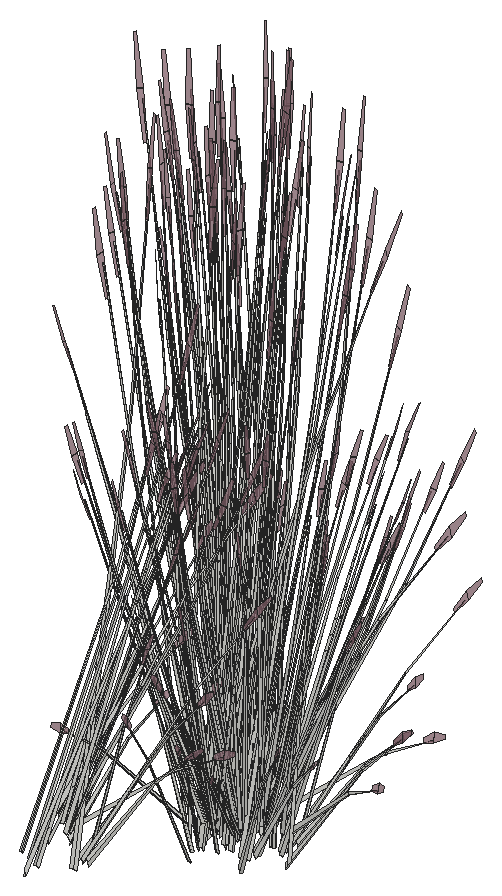
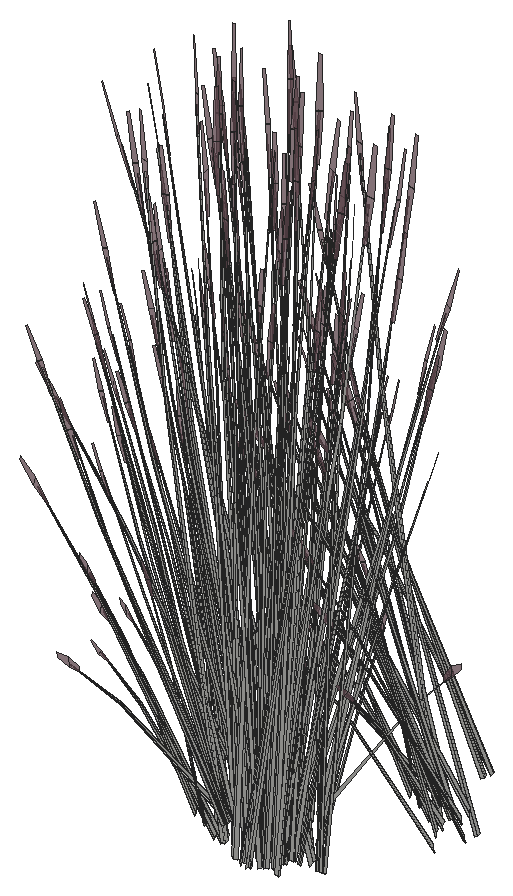
# SketchUp Ruby script. Lengths in inches.
U = 1.inch
M = Sketchup.active_model
def pt(a) = Geom::Point3d.new(a.map { |v| v * U })
def face(e, loops, mat)
  f = e.add_face(loops[0].map { |a| pt(a) })
  loops[1..].each { |l| e.add_face(l.map { |a| pt(a) }).erase! }
  f.material = f.back_material = mat if mat
  f
end
# faces: each face lists its corners as indices into pts; further lists are holes
def faces(e, pts, list, mat = nil) = list.each { |f| face(e, (f[0].is_a?(Array) ? f : [f]).map { |l| l.map { |i| pts[i] } }, mat) }
# xy, xz, yz: faces in a plane at the given z, y or x. An outline is a flat list of corners, or four numbers for a rectangle; further outlines are holes
def ring(l) = l.size == 4 ? [[l[0], l[1]], [l[2], l[1]], [l[2], l[3]], [l[0], l[3]]] : l.each_slice(2).to_a
def flat(e, list, mat, &to3) = list.each { |f| face(e, (f[0].is_a?(Array) ? f : [f]).map { |l| ring(l).map { |u, v| to3.(u, v) } }, mat) }
def xy(e, z, list, mat = nil) = flat(e, list, mat) { |x, y| [x, y, z] }
def xz(e, y, list, mat = nil) = flat(e, list, mat) { |x, z| [x, y, z] }
def yz(e, x, list, mat = nil) = flat(e, list, mat) { |y, z| [x, y, z] }
def lines(e, pts, list) = list.each { |a, b| e.add_line(pt(pts[a]), pt(pts[b])) }
# prism: a flat outline (further loops are holes) pulled along v
def prism(e, loops, v, mat = nil)
  f = face(e, loops, mat); d = Geom::Vector3d.new(v.map { |x| x * U })
  f.pushpull(f.normal.samedirection?(d) ? d.length : -d.length)
end
def box(e, o, s, mat = nil) = prism(e, [[o, [o[0] + s[0], o[1], o[2]], [o[0] + s[0], o[1] + s[1], o[2]], [o[0], o[1] + s[1], o[2]]]], [0, 0, s[2]], mat)
def at(x, y, z, deg = 0) = Geom::Transformation.translation(pt([x, y, z])) * Geom::Transformation.rotation(ORIGIN, Z_AXIS, deg.degrees)
def axes(o, x, y, z) = Geom::Transformation.new([*x, 0, *y, 0, *z, 0, *pt(o).to_a, 1])
def part(name) = M.definitions.add(name)
# library, detail: a bought-in or finely detailed component or shape, given as its bounding box
def library(name, o, s) = part(name).tap { |d| box(d.entities, o, s) }
def detail(e, o, s) = box(e.add_group.entities, o, s)
def put(e, d, t, mat = nil) = e.add_instance(d, t).tap { |i| i.material = mat if mat }
def group(e, t, mat = nil) = e.add_group.tap { |g| g.transformation = t; g.material = mat if mat }.entities
root = M.entities
M.materials.add("LightPink_Translucent").color = [144, 107, 117]
M.materials["LightPink_Translucent"].alpha = 0.75
c1 = part("blade")
p = [[2.15,0.21,22],[0,0.17,0],[0.09,0.45,0],[2.18,0.31,22],[2.29,0.31,22],[0.38,0.45,0],
  [2.48,0.24,33],[2.49,0.24,33],[2.48,0.22,33]]
faces(c1.entities,p,[[0,1,2,3],[4,5,2,3],[6,3,4,7],[8,0,3,6]])
c2 = part("seeds")
p = [[0.3,-0.1,1.38],[-0.01,-0.03,1.59],[-0.01,-0.03,0.03],[0.14,-0.07,-0.07],[0.29,-0.03,3],[0.15,0.01,3.11]]
faces(c2.entities,p,[[0,1,2,3],[1,0,4,5]],"LightPink_Translucent")
c3 = part("blade with seeds")
put(c3.entities,c1,at(0,0,0))
put(c3.entities,c2,axes([2.4,0.25,30.99],[1.5799,-0.05474,1.17369],[-0.12525,1.92788,0.29478],[-0.07173,-0.02425,1.56792]))
put(root,c3,axes([292.125,487.27,4.73],[0.32857,0.44488,0.0643],[-0.59916,0.21775,0.50621],[0.26412,-0.04296,0.77189]))
put(root,c3,axes([292.0625,487.11,4.73],[-0.25275,0.59491,0.48003],[-0.83094,-0.20343,0.3958],[0.32677,-0.03575,0.9933]))
put(root,c3,axes([291.625,482.97,4.68],[0.87941,0.16356,-0.51099],[-0.30143,0.56078,-0.3958],[0.08064,0.22578,0.97773]))
put(root,c3,axes([292.12,481.81,3.875],[-0.2045,-0.20949,1.71376],[0.94495,-0.17636,0.13857],[0.21357,0.32887,0.73262]))
put(root,c3,axes([289.7,486,2.06],[0.9306,0.10697,-0.62353],[-0.19638,0.65984,-0.16365],[0.27771,0.07995,1.37633]))
put(root,c3,axes([293.81,487.15,2.77],[-0.55274,0.10771,1.1486],[0.26018,-0.44517,0.84392],[0.29323,0.03046,0.25299]))
put(root,c3,axes([293.55,489.04,4.71],[-0.08089,-0.05712,1.77383],[0.17695,-0.61228,-0.16761],[0.31864,-0.03912,0.31391]))
put(root,c3,axes([291.3,482.86,4.98],[0.42698,0.53052,-0.71045],[-0.87893,0.29566,0.08574],[0.09984,0.25633,1.00501]))
put(root,c3,axes([292.85,488.53,3.93],[-0.17122,-0.54847,-0.03492],[0.80929,-0.12609,-0.15832],[0.169,0.03477,0.52218]))
put(root,c3,axes([290.75,488.51,5.03],[0.0479,-0.66354,-0.1216],[0.90696,0.01814,-0.67495],[0.3493,0.04609,1.02557]))
put(root,c3,axes([290.61,488.25,5.05],[-0.50902,-0.40851,0.35414],[0.58122,-0.38671,-0.4572],[0.29531,0.05884,0.87481]))
put(root,c3,axes([292.77,487.87,2.59],[-0.21545,-0.16047,1.43002],[0.28033,-0.53085,-0.30754],[0.43591,0.07191,0.61141]))
put(root,c3,axes([291.54,488.11,4.72],[0.19191,-0.01103,1.74944],[0.52639,-0.5069,-0.27667],[0.34136,0.06691,0.14031]))
put(root,c3,axes([290.8,488.19,4.98],[0.89428,0.01571,-0.71045],[-0.06006,0.66153,0.08574],[0.37886,0.06981,1.00501]))
put(root,c3,axes([297.4,493.71,4.72],[-0.13683,-0.09148,1.74944],[-0.91315,0.058,-0.27667],[-0.14574,-0.2188,0.14031]))
put(root,c3,axes([299.52,494.8,2.59],[-0.25429,0.13207,1.43002],[-0.76157,-0.23115,-0.30754],[0.14117,-0.28747,0.61141]))
put(root,c3,axes([298.36,495.26,4.98],[-0.42698,-0.53052,-0.71045],[0.87893,-0.29566,0.08574],[-0.09984,-0.25633,1.00501]))
put(root,c3,axes([292.26,486.85,2.375],[1.11865,0,0],[0,0.72922,-0.51607],[0,0.16609,1.63711]))
put(root,c3,axes([297.62,494.08,1.49],[-0.15005,0.02351,1.76342],[-0.82981,-0.26461,-0.26939],[0.01392,-0.22072,0.30037]))
put(root,c3,axes([291.33,488.46,4.53],[0.50902,0.40851,-0.35414],[-0.58122,0.38671,0.4572],[0.29531,0.05884,0.87481]))
put(root,c3,axes([291.07,488.62,4.73],[-0.04505,0.49615,0.0643],[-0.68022,-0.0136,0.50621],[0.26056,0.05192,0.77189]))
put(root,c3,axes([300.14,495.77,4.98],[0.02328,-0.60353,-0.71045],[0.98022,0.04053,0.08574],[0.10344,-0.25568,1.00501]))
put(root,c3,axes([291.14,488.46,4.73],[-0.65964,0.42992,0.48003],[-0.5689,-0.45657,0.3958],[0.30948,0.0793,0.9933]))
put(root,c3,axes([301.5,494.83,4.72],[-0.00864,-0.12985,1.74944],[-0.72937,-0.3753,-0.27667],[0.11277,-0.2275,0.14031]))
put(root,c3,axes([298.44,494.8,4.53],[0.2697,-0.50175,-0.35414],[0.78684,0.14635,0.4572],[-0.07215,-0.20201,0.87481]))
put(root,c3,axes([299.03,495.47,3.875],[-0.16657,0.22426,1.71376],[-0.69879,-0.4641,0.13857],[0.31524,-0.28926,0.73262]))
put(root,c3,axes([301.31,494.37,4.71],[-0.09085,0.04984,1.77383],[-0.89014,-0.16814,-0.16761],[-0.03222,-0.21748,0.31391]))
put(root,c3,axes([298.04,495.15,4.68],[-0.87941,-0.16356,-0.51099],[0.30143,-0.56078,-0.3958],[-0.08064,-0.22578,0.97773]))
put(root,c3,axes([298.58,493.74,2.77],[0.11476,0.38047,1.1486],[-0.63664,-0.21072,0.84392],[0.06851,-0.19481,0.25299]))
put(root,c3,axes([299.9375,495.57,4.68],[-0.64041,-0.4384,-0.51099],[0.67652,-0.38394,-0.3958],[0.09744,-0.22274,0.97773]))
put(root,c3,axes([289.51,487.42,3.875],[-0.3323,-0.11241,1.71376],[0.68769,-0.4716,0.13857],[0.42861,0.21275,0.73262]))
put(root,c3,axes([296.28,494.8,5.09],[0.99656,-0.1677,0.53763],[0.17295,0.65785,0.4433],[-0.23438,-0.19388,1.11249]))
put(root,c3,axes([298.54,494.92,4.73],[0.88151,0.17057,0.48003],[-0.30143,0.56078,0.3958],[-0.05297,-0.22053,0.9933]))
put(root,c3,axes([290.74,488.7,2.77],[-0.5037,-0.18761,1.1486],[0.6504,-0.19062,0.84392],[0.17543,0.16147,0.25299]))
put(root,c3,axes([298.79,495.12,5.03],[-0.87543,0.30377,-0.1216],[-0.4302,-0.53915,-0.67495],[-0.1155,-0.2272,1.02557]))
put(root,c3,axes([288.97,489.23,5.03],[0.53309,-0.55848,-0.1216],[0.77201,0.32175,-0.67495],[0.26836,0.15779,1.02557]))
put(root,c3,axes([300.61,495.8,5.03],[-0.98321,-0.03233,-0.1216],[0.02687,-0.61208,-0.67495],[0.0683,-0.23574,1.02557]))
put(root,c3,axes([300.54,495.41,4.53],[0.60531,-0.34352,-0.35414],[0.573,0.39225,0.4572],[0.08718,-0.19929,0.87481]))
put(root,c3,axes([298.77,494.88,4.73],[0.6592,-0.22175,0.0643],[0.32265,0.40436,0.50621],[-0.06366,-0.17825,0.77189]))
put(root,c3,axes([288.27,489.7,4.71],[0.00265,-0.07899,1.77383],[0.76665,-0.34851,-0.16761],[0.2663,0.12439,0.31391]))
put(root,c3,axes([290.88,489.39,1.49],[0.06518,-0.0942,1.76342],[0.82057,-0.27742,-0.26939],[0.24877,0.14358,0.30037]))
put(root,c3,axes([289.6,488.95,4.68],[0.88277,-0.1551,-0.51099],[0.15442,0.58737,-0.3958],[0.23711,0.16832,0.97773]))
put(root,c3,axes([296.51,494.94,4.73],[0.4066,-0.41448,0.0643],[0.57901,0.24131,0.50621],[-0.18719,-0.13288,0.77189]))
put(root,c3,axes([296.38,497.25,2.1],[-0.36739,-0.66907,-0.69835],[1.05831,-0.24096,-0.18329],[-0.04061,-0.22656,1.54149]))
put(root,c3,axes([301.3,495.2,1.49],[-0.1339,-0.0514,1.76342],[-0.34394,-0.57425,-0.26939],[0.23202,-0.15583,0.30037]))
put(root,c3,axes([290.82,489.55,2.67],[-0.57368,-0.02046,1.0506],[0.37886,-0.43461,0.58006],[0.22663,0.15441,0.8241]))
put(root,c3,axes([298.53,495.33,5.05],[-0.2697,0.50175,0.35414],[-0.78684,-0.14635,-0.4572],[-0.07215,-0.20201,0.87481]))
put(root,c3,axes([300.54,495.54,4.73],[0.63704,0.44518,0.48003],[-0.67652,0.38394,0.3958],[0.11751,-0.20886,0.9933]))
put(root,c3,axes([300.77,495.59,4.73],[0.73517,0.0304,0.0643],[-0.02016,0.45906,0.50621],[0.07693,-0.17585,0.77189]))
put(root,c3,axes([300.22,495.9,5.05],[-0.60531,0.34352,0.35414],[-0.573,-0.39225,-0.4572],[0.08718,-0.19929,0.87481]))
put(root,c3,axes([301.29,496.82,4.98],[0.4673,-0.51481,-0.71045],[0.81887,0.36587,0.08574],[0.27902,-0.18652,1.00501]))
put(root,c3,axes([296.24,495.32,2.375],[-0.55932,-0.6538,0],[0.93577,-0.36461,-0.51607],[0.21313,-0.08304,1.63711]))
put(root,c3,axes([301.27,496.58,4.68],[-0.22982,-0.59576,-0.51099],[0.87033,-0.10422,-0.3958],[0.24941,-0.16002,0.97773]))
put(root,c3,axes([288.94,488.5,2.59],[0.01579,-0.21629,1.43002],[0.75442,-0.24159,-0.30754],[0.23289,0.25887,0.61141]))
put(root,c3,axes([297.47,494.54,2.13],[-0.61821,0.37431,-0.03893],[-0.56645,-0.40995,-0.17649],[-0.03988,-0.11616,0.58215]))
put(root,c3,axes([301.68,497.01,5.03],[-0.82753,-0.35977,-0.1216],[0.47675,-0.52101,-0.67495],[0.2338,-0.18111,1.02557]))
put(root,c3,axes([294.22,497.15,2.02],[0,-0.65246,-0.49651],[1.00089,0,0],[0,-0.1486,1.57504]))
put(root,c3,axes([297,495.22,2.02],[0.83726,-0.32623,-0.49651],[0.50045,0.58498,0],[0.19069,-0.0743,1.57504]))
put(root,c3,axes([301.97,496.35,2.59],[-0.31959,-0.01933,1.43002],[-0.32741,-0.51843,-0.30754],[0.39262,-0.14666,0.61141]))
put(root,c3,axes([303.72,496.85,4.71],[-0.11685,-0.00496,1.77383],[-0.48522,-0.53096,-0.16761],[0.19486,-0.17458,0.31391]))
put(root,c3,axes([297.99,496.5625,2.06],[0.60257,-0.49041,-0.62353],[0.74854,0.44469,-0.16365],[0.24146,-0.12234,1.37633]))
put(root,c3,axes([302.34,495.4,2.77],[-0.29798,0.33213,1.1486],[-0.25612,-0.44624,0.84392],[0.24611,-0.11182,0.25299]))
put(root,c3,axes([301.91,496.65,4.53],[0.77872,-0.09325,-0.35414],[0.20563,0.53305,0.4572],[0.22316,-0.14318,0.87481]))
put(root,c3,axes([296.94,497.42,2.21],[0.43405,-0.58792,-0.44739],[0.90188,0.28295,0.21531],[0,-0.13553,1.43643]))
put(root,c3,axes([297.34,497.13,2.67],[-0.10425,-0.7445,-0.29095],[1.08575,-0.04502,-0.50002],[0.19119,-0.09917,1.59708]))
put(root,c3,axes([294.65,497.17,2.03],[0.62448,-0.40708,-0.30978],[0.62448,0.40708,0.30978],[0,-0.13112,1.38974]))
put(root,c3,axes([301.28,496.96,5.05],[-0.77872,0.09325,0.35414],[-0.20563,-0.53305,-0.4572],[0.22316,-0.14318,0.87481]))
put(root,c3,axes([296.83,497.91,2.67],[-1.00749,-0.31132,-0.29095],[0.48511,-0.65709,-0.50002],[-0.03166,-0.16133,1.59708]))
put(root,c3,axes([297.2,495.48,2.03],[0.83462,0.16144,-0.30978],[-0.21015,0.56852,0.30978],[0.16826,-0.06556,1.38974]))
put(root,c3,axes([301.98,496.875,4.73],[0.61415,0.2744,0.0643],[-0.35756,0.39076,0.50621],[0.1969,-0.12633,0.77189]))
put(root,c3,axes([301.81,496.76,4.73],[0.22187,0.60049,0.48003],[-0.87033,0.10422,0.3958],[0.25651,-0.14123,0.9933]))
put(root,c3,axes([304.16,497.49,4.72],[0.12414,-0.09938,1.74944],[-0.15889,-0.60963,-0.27667],[0.31148,-0.11559,0.14031]))
put(root,c3,axes([297.48,497.71,2.43],[1.00799,0.31623,0.24065],[-0.48511,0.65709,0.50002],[0,-0.15147,1.60543]))
put(root,c3,axes([297.09,498.6,2.4375],[0.23711,-0.77313,-0.23429],[1.12425,0.13477,0.51271],[-0.19645,-0.10677,1.5644]))
put(root,c3,axes([297.16,497.27,2.72],[-0.97146,0.04028,0.44739],[-0.08785,-0.66859,-0.21531],[0.17391,-0.06776,1.43643]))
put(root,c3,axes([294.65,497.76,2.48],[0,0.65246,0.49651],[-1.00089,0,0],[0,-0.1486,1.57504]))
put(root,c3,axes([301.71,498.41,5.03],[-0.45012,-0.59081,-0.1216],[0.79888,-0.29033,-0.67495],[0.33665,-0.07795,1.02557]))
put(root,c3,axes([301.67,497.91,4.68],[0.24236,-0.59349,-0.51099],[0.83094,0.20343,-0.3958],[0.33455,-0.05442,0.97773]))
put(root,c3,axes([300.36,495.49,2.375],[0.55932,-0.6538,0],[0.93577,0.36461,-0.51607],[0.21313,0.08304,1.63711]))
put(root,c3,axes([297.01,498.29,2.21],[-0.53742,-0.54764,-0.44739],[0.81403,-0.38564,0.21531],[-0.17391,-0.06776,1.43643]))
put(root,c3,axes([297.12,497.51,2.36],[0.38895,0.72959,0.45755],[-1.11135,0.2537,0.17955],[0.01358,-0.13406,1.58856]))
put(root,c3,axes([302.5625,498.07,1.98],[-0.57619,0.0783,1.41583],[-0.09171,-0.62326,0.08104],[0.40356,-0.09434,0.80566]))
put(root,c3,axes([303.61,497.52,2.26],[-0.55463,-0.41721,-0.06488],[0.60744,-0.38228,-0.29416],[0.17212,-0.02691,0.97024]))
put(root,c3,axes([296.93,498.09,2.72],[-0.43405,0.58792,0.44739],[-0.90188,-0.28295,-0.21531],[0,-0.13553,1.43643]))
put(root,c3,axes([298.52,497.58,2.21],[0,-0.75495,0],[1.11865,0,0],[0,0,1.79456]))
put(root,c3,axes([299.875,495.83,2.48],[-0.83726,-0.32623,0.49651],[0.50045,-0.58498,0],[0.19069,0.0743,1.57504]))
put(root,c3,axes([301.51,498.12,4.98],[0.78611,-0.28816,-0.71045],[0.4381,0.59317,0.08574],[0.37982,-0.06738,1.00501]))
put(root,c3,axes([297.99,497.1,2.36],[-0.74176,0.59212,0.45755],[-0.88124,-0.52269,0.17955],[0.17882,-0.05909,1.58856]))
put(root,c3,axes([298.8,498.16,2.3],[-0.83213,-0.56158,-0.06131],[0.83263,-0.56193,0],[-0.02906,-0.01961,1.75571]))
put(root,c3,axes([296.7,496.125,2.47],[-0.25843,0.64844,0.17642],[-0.9457,-0.1835,0.35086],[0.16336,-0.00316,1.60407]))
put(root,c3,axes([301.4,498.24,5.05],[-0.74348,-0.18202,0.35414],[0.21685,-0.53102,-0.4572],[0.29933,-0.04869,0.87481]))
put(root,c3,axes([296.3125,496.65,1.59],[-0.88056,0.26122,1.28929],[-0.28027,-0.74951,0.50096],[0.54072,0.01247,1.46642]))
put(root,c3,axes([298.68,496.85,2.62],[0.17258,-0.58229,0.1448],[0.84319,0.10108,-0.41347],[0.15345,0.05979,1.26744]))
put(root,c3,axes([297.22,498.23,2.36],[1.13071,0.13747,0.45755],[-0.23011,0.77639,0.17955],[-0.16524,-0.07497,1.58856]))
put(root,c3,axes([303.1875,497.67,1.49],[-0.04675,-0.09906,1.76342],[0.32428,-0.57943,-0.26939],[0.32711,-0.00833,0.30037]))
put(root,c3,axes([298.32,497,2.72],[-0.53742,-0.54764,0.44739],[0.81403,-0.38564,-0.21531],[0.17391,0.06776,1.43643]))
put(root,c3,axes([296.61,499.47,2.47],[0.96132,-0.17317,0.17642],[0.23737,0.64447,0.35086],[-0.08574,-0.0939,1.60407]))
put(root,c3,axes([298.59,497.03,2.67],[0.90324,-0.43318,-0.29095],[0.60064,0.61207,-0.50002],[0.22285,0.06216,1.59708]))
put(root,c3,axes([302.18,498.18,4.53],[0.74348,0.18202,-0.35414],[-0.21685,0.53102,0.4572],[0.29933,-0.04869,0.87481]))
put(root,c3,axes([300.87,495.88,2.02],[0.83726,0.32623,-0.49651],[-0.50045,0.58498,0],[0.19069,0.0743,1.57504]))
put(root,c3,axes([299.28,497.74,2.21],[1.00089,0,0],[0,0.67548,0],[0,0,1.78407]))
put(root,c3,axes([299.5625,496.16,2.47],[-0.96132,0.17317,0.17642],[-0.23737,-0.64447,0.35086],[0.08574,0.0939,1.60407]))
put(root,c3,axes([300.16,497.52,3.875],[-0.37107,0.01478,1.71376],[0.24616,-0.64047,0.13857],[0.5288,0.03961,0.73262]))
put(root,c3,axes([300.64,496.125,2.03],[0.21015,0.56852,-0.30978],[-0.83462,0.16144,0.30978],[0.16826,0.06556,1.38974]))
put(root,c3,axes([302.07,498.4,4.73],[0.32857,0.44488,0.0643],[-0.59916,0.21775,0.50621],[0.26412,-0.04296,0.77189]))
put(root,c3,axes([298.96,497.4,2.38],[-1.13071,-0.13747,0.49198],[0.23011,-0.77639,0.19306],[0.16524,0.07497,1.70813]))
put(root,c3,axes([302.01,498.24,4.73],[-0.25275,0.59491,0.48003],[-0.83094,-0.20343,0.3958],[0.32677,-0.03575,0.9933]))
put(root,c3,axes([298.05,499.32,2.2],[-0.29189,-0.56252,0],[0.83351,-0.19699,0],[0,0,1.54371]))
put(root,c3,axes([297.5,498.78,2.62],[-0.17258,0.58229,0.1448],[-0.84319,-0.10108,-0.41347],[-0.15345,-0.05979,1.26744]))
put(root,c3,axes([299.15,499.24,2.18],[0.93921,-0.22138,-0.19198],[0.33003,0.6377,0.00008],[0.10367,-0.02447,1.73897]))
put(root,c3,axes([299.47,499.5,2.47],[0.25843,-0.64844,0.17642],[0.9457,0.1835,0.35086],[-0.16336,0.00316,1.60407]))
put(root,c3,axes([299.26,498.03,2.21],[0.62448,0.42144,0],[-0.62448,0.42144,0],[0,0,1.69266]))
put(root,c3,axes([300.95,497.85,2.47],[-0.70288,-0.47526,0.17642],[0.70832,-0.46097,0.35086],[-0.07763,0.09706,1.60407]))
put(root,c3,axes([299.65,497.13,2.06],[0.9306,0.10697,-0.62353],[-0.19638,0.65984,-0.16365],[0.27771,0.07995,1.37633]))
put(root,c3,axes([303.76,498.28,2.77],[-0.55274,0.10771,1.1486],[0.26018,-0.44517,0.84392],[0.29323,0.03046,0.25299]))
put(root,c3,axes([297.85,499.57,2.2],[-0.90188,-0.29293,0],[0.43405,-0.60866,0],[0,0,1.62707]))
put(root,c3,axes([298.6,498.79,2.46],[-0.87356,-0.52515,-0.25192],[0.73507,-0.5897,0.5513],[-0.23523,0.06143,1.68216]))
put(root,c3,axes([296.3,499.8,2.48],[0.83726,0.32623,0.49651],[-0.50045,0.58498,0],[-0.19069,-0.0743,1.57504]))
put(root,c3,axes([299.25,497.54,2.72],[0.43405,-0.58792,0.44739],[0.90188,0.28295,-0.21531],[0,0.13553,1.43643]))
put(root,c3,axes([303.5,500.17,4.71],[-0.08089,-0.05712,1.77383],[0.17695,-0.61228,-0.16761],[0.31864,-0.03912,0.31391]))
put(root,c3,axes([299.08,497.875,2.29],[0,0.75458,-0.05637],[-1.11865,0,0],[0,0.02371,1.79368]))
put(root,c3,axes([299.16,497.34,2.21],[0.53742,0.54764,-0.44739],[-0.81403,0.38564,0.21531],[0.17391,0.06776,1.43643]))
put(root,c3,axes([302.8,499.66,3.93],[-0.17122,-0.54847,-0.03492],[0.80929,-0.12609,-0.15832],[0.169,0.03477,0.52218]))
put(root,c3,axes([300.7,499.64,5.03],[0.0479,-0.66354,-0.1216],[0.90696,0.01814,-0.67495],[0.3493,0.04609,1.02557]))
put(root,c3,axes([301.53,497.87,2.48],[0,-0.65246,0.49651],[1.00089,0,0],[0,0.1486,1.57504]))
put(root,c3,axes([299.02,498.36,2.72],[0.97146,-0.04028,0.44739],[0.08785,0.66859,-0.21531],[-0.17391,0.06776,1.43643]))
put(root,c3,axes([299.625,497.67,2.62],[0.83351,-0.19028,0.1448],[0.29189,0.54335,-0.41347],[0,0.11958,1.26744]))
put(root,c3,axes([300.5625,499.38,5.05],[-0.50902,-0.40851,0.35414],[0.58122,-0.38671,-0.4572],[0.29531,0.05884,0.87481]))
put(root,c3,axes([298.16,498.68,2.21],[-0.97146,0.04028,-0.44739],[-0.08785,-0.66859,0.21531],[-0.17391,0.06776,1.43643]))
put(root,c3,axes([302.72,499,2.59],[-0.21545,-0.16047,1.43002],[0.28033,-0.53085,-0.30754],[0.43591,0.07191,0.61141]))
put(root,c3,axes([298.87,499.58,2.2],[0.90188,0.29293,0],[-0.43405,0.60866,0],[0,0,1.74954]))
put(root,c3,axes([301.49,499.24,4.72],[0.19191,-0.01103,1.74944],[0.52639,-0.5069,-0.27667],[0.34136,0.06691,0.14031]))
put(root,c3,axes([299.23,500.23,2.19],[-0.55235,-0.65609,-0.05142],[0.93577,-0.36461,0.51607],[-0.23059,0.06247,1.6363]))
put(root,c3,axes([299.04,498.64,2.62],[0.66093,0.39201,0.1448],[-0.5513,0.44227,-0.41347],[-0.15345,0.05979,1.26744]))
put(root,c3,axes([300.75,499.32,4.98],[0.89428,0.01571,-0.71045],[-0.06006,0.66153,0.08574],[0.37886,0.06981,1.00501]))
put(root,c3,axes([299.74,499.85,2.48],[0.83726,-0.32623,0.49651],[0.50045,0.58498,0],[-0.19069,0.0743,1.57504]))
put(root,c3,axes([298.55,499.34,2.29],[0.38895,0.74956,-0.06012],[-1.11135,0.26265,0],[0.01358,0.02618,1.72173]))
put(root,c3,axes([298.98,500.15,2.03],[-0.83462,-0.16144,-0.30978],[0.21015,-0.56852,0.30978],[-0.16826,0.06556,1.38974]))
put(root,c3,axes([302.21,497.98,2.375],[1.11865,0,0],[0,0.72922,-0.51607],[0,0.16609,1.63711]))
put(root,c3,axes([301.76,498.35,2.2],[-1.1181,-0.00522,-0.04976],[0,-0.72922,0.49943],[-0.03514,0.166,1.58352]))
put(root,c3,axes([299.34,497.72,2.67],[1.00749,0.31132,-0.29095],[-0.48511,0.65709,-0.50002],[0.03166,0.16133,1.59708]))
put(root,c3,axes([301.28,499.59,4.53],[0.50902,0.40851,-0.35414],[-0.58122,0.38671,0.4572],[0.29531,0.05884,0.87481]))
put(root,c3,axes([301.53,498.46,2.03],[-0.62448,0.40708,-0.30978],[-0.62448,-0.40708,0.30978],[0,0.13112,1.38974]))
put(root,c3,axes([298.84,498.5,2.67],[0.10425,0.7445,-0.29095],[-1.08575,0.04502,-0.50002],[-0.19119,0.09917,1.59708]))
put(root,c3,axes([301.02,499.75,4.73],[-0.04505,0.49615,0.0643],[-0.68022,-0.0136,0.50621],[0.26056,0.05192,0.77189]))
